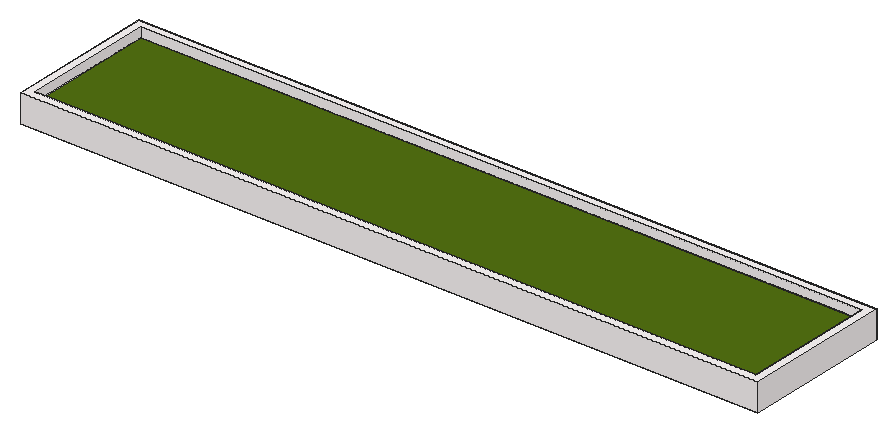
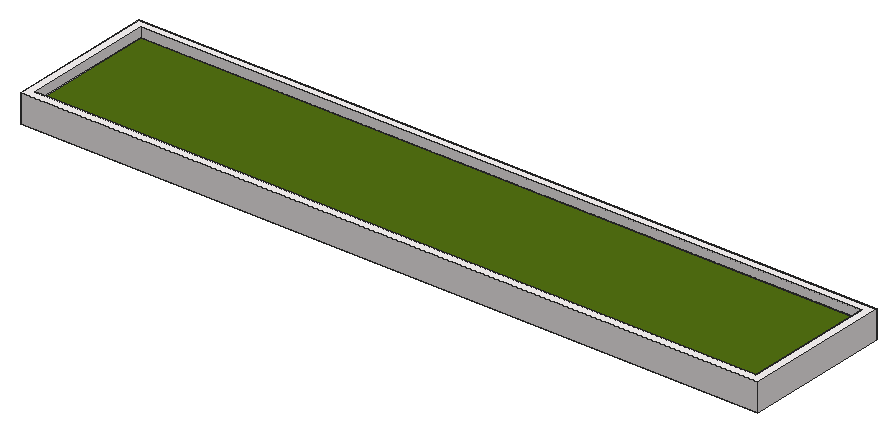
# SketchUp Ruby script. Lengths in inches.
U = 1.inch
M = Sketchup.active_model
def pt(a) = Geom::Point3d.new(a.map { |v| v * U })
def face(e, loops, mat)
  f = e.add_face(loops[0].map { |a| pt(a) })
  loops[1..].each { |l| e.add_face(l.map { |a| pt(a) }).erase! }
  f.material = f.back_material = mat if mat
  f
end
# faces: each face lists its corners as indices into pts; further lists are holes
def faces(e, pts, list, mat = nil) = list.each { |f| face(e, (f[0].is_a?(Array) ? f : [f]).map { |l| l.map { |i| pts[i] } }, mat) }
# xy, xz, yz: faces in a plane at the given z, y or x. An outline is a flat list of corners, or four numbers for a rectangle; further outlines are holes
def ring(l) = l.size == 4 ? [[l[0], l[1]], [l[2], l[1]], [l[2], l[3]], [l[0], l[3]]] : l.each_slice(2).to_a
def flat(e, list, mat, &to3) = list.each { |f| face(e, (f[0].is_a?(Array) ? f : [f]).map { |l| ring(l).map { |u, v| to3.(u, v) } }, mat) }
def xy(e, z, list, mat = nil) = flat(e, list, mat) { |x, y| [x, y, z] }
def xz(e, y, list, mat = nil) = flat(e, list, mat) { |x, z| [x, y, z] }
def yz(e, x, list, mat = nil) = flat(e, list, mat) { |y, z| [x, y, z] }
def lines(e, pts, list) = list.each { |a, b| e.add_line(pt(pts[a]), pt(pts[b])) }
# prism: a flat outline (further loops are holes) pulled along v
def prism(e, loops, v, mat = nil)
  f = face(e, loops, mat); d = Geom::Vector3d.new(v.map { |x| x * U })
  f.pushpull(f.normal.samedirection?(d) ? d.length : -d.length)
end
def box(e, o, s, mat = nil) = prism(e, [[o, [o[0] + s[0], o[1], o[2]], [o[0] + s[0], o[1] + s[1], o[2]], [o[0], o[1] + s[1], o[2]]]], [0, 0, s[2]], mat)
def at(x, y, z, deg = 0) = Geom::Transformation.translation(pt([x, y, z])) * Geom::Transformation.rotation(ORIGIN, Z_AXIS, deg.degrees)
def axes(o, x, y, z) = Geom::Transformation.new([*x, 0, *y, 0, *z, 0, *pt(o).to_a, 1])
def part(name) = M.definitions.add(name)
# library, detail: a bought-in or finely detailed component or shape, given as its bounding box
def library(name, o, s) = part(name).tap { |d| box(d.entities, o, s) }
def detail(e, o, s) = box(e.add_group.entities, o, s)
def put(e, d, t, mat = nil) = e.add_instance(d, t).tap { |i| i.material = mat if mat }
def group(e, t, mat = nil) = e.add_group.tap { |g| g.transformation = t; g.material = mat if mat }.entities
root = M.entities
M.materials.add("[0010_Snow]").color = [255, 250, 250]
M.materials.add("[Vegetation_Blur7]").color = [83, 114, 18]
xy(root,0,[[208.39,63.73,375.84,94.42]])
xy(root,0,[[[206.42,61.9,377.8125,96.24],[208.39,63.73,375.84,94.42]]],"[0010_Snow]")
xy(root,4.31,[[208.39,63.73,375.84,94.42]],"[Vegetation_Blur7]")
xy(root,6.46,[[[206.42,61.9,377.8125,96.24],[208.39,63.73,375.84,94.42]]],"[0010_Snow]")
xz(root,61.9,[[206.42,0,377.8125,6.46]],"[0010_Snow]")
xz(root,63.73,[[208.39,0,375.84,4.31],[208.39,4.31,375.84,6.46]],"[0010_Snow]")
xz(root,94.42,[[208.39,0,375.84,4.31],[208.39,4.31,375.84,6.46]],"[0010_Snow]")
xz(root,96.24,[[206.42,0,377.8125,6.46]],"[0010_Snow]")
yz(root,206.42,[[61.9,0,96.24,6.46]],"[0010_Snow]")
yz(root,208.39,[[63.73,0,94.42,4.31],[63.73,4.31,94.42,6.46]],"[0010_Snow]")
yz(root,375.84,[[63.73,0,94.42,4.31],[63.73,4.31,94.42,6.46]],"[0010_Snow]")
yz(root,377.8125,[[61.9,0,96.24,6.46]],"[0010_Snow]")
